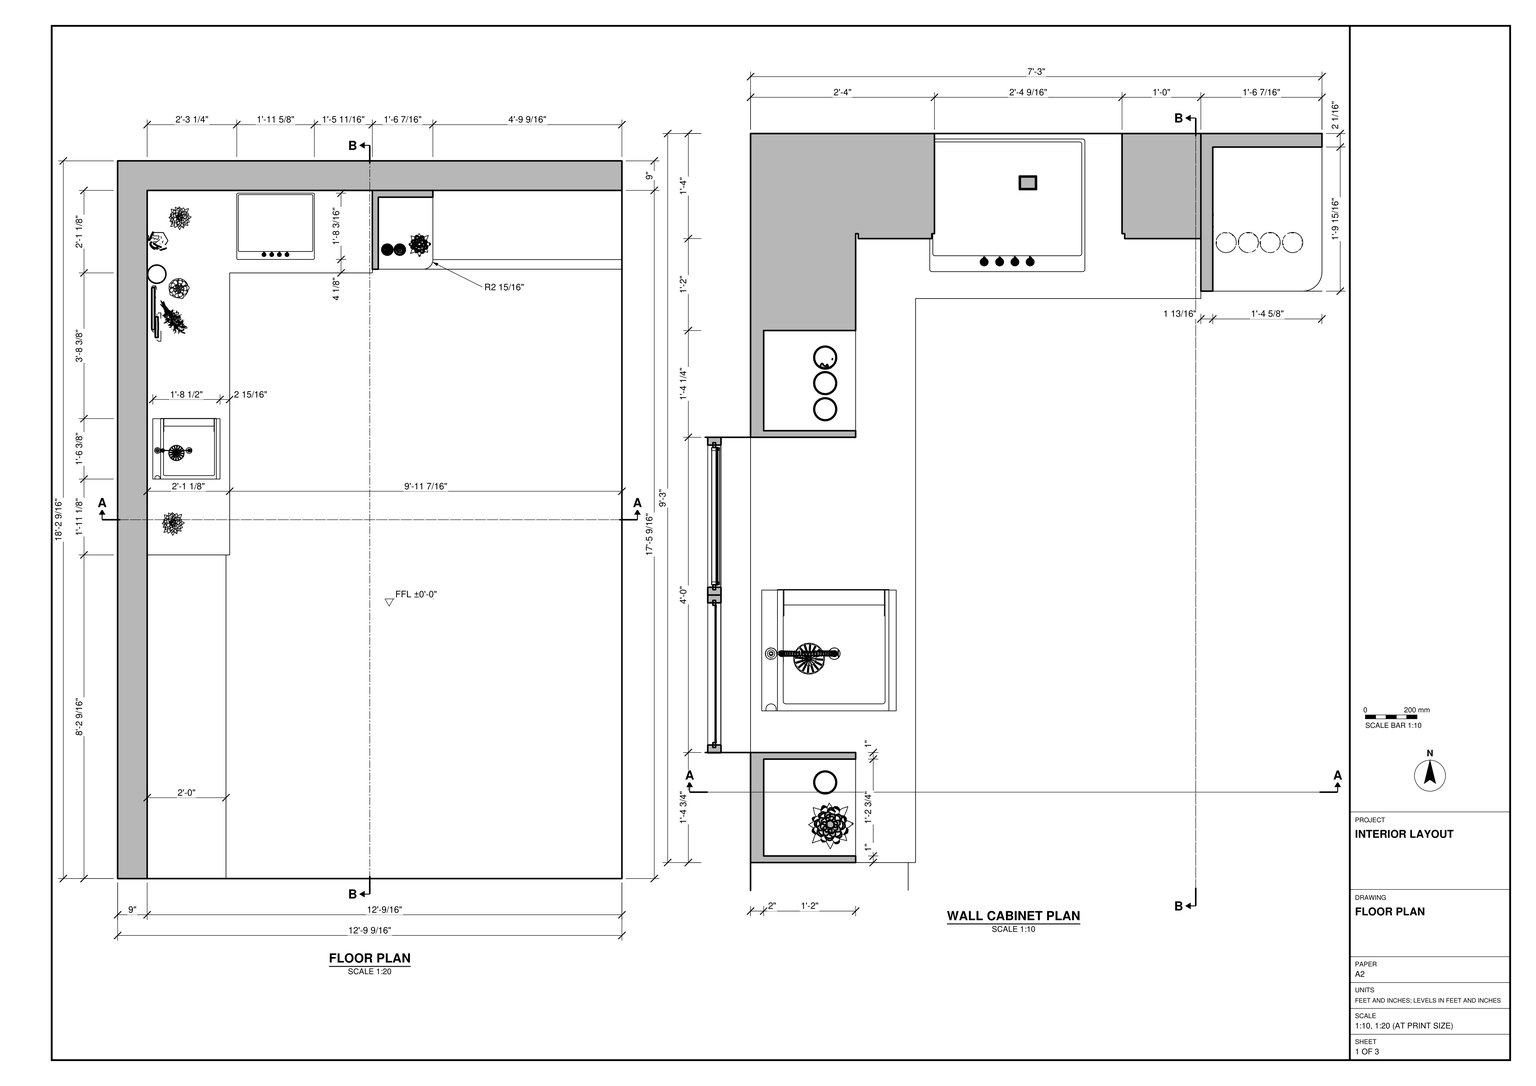
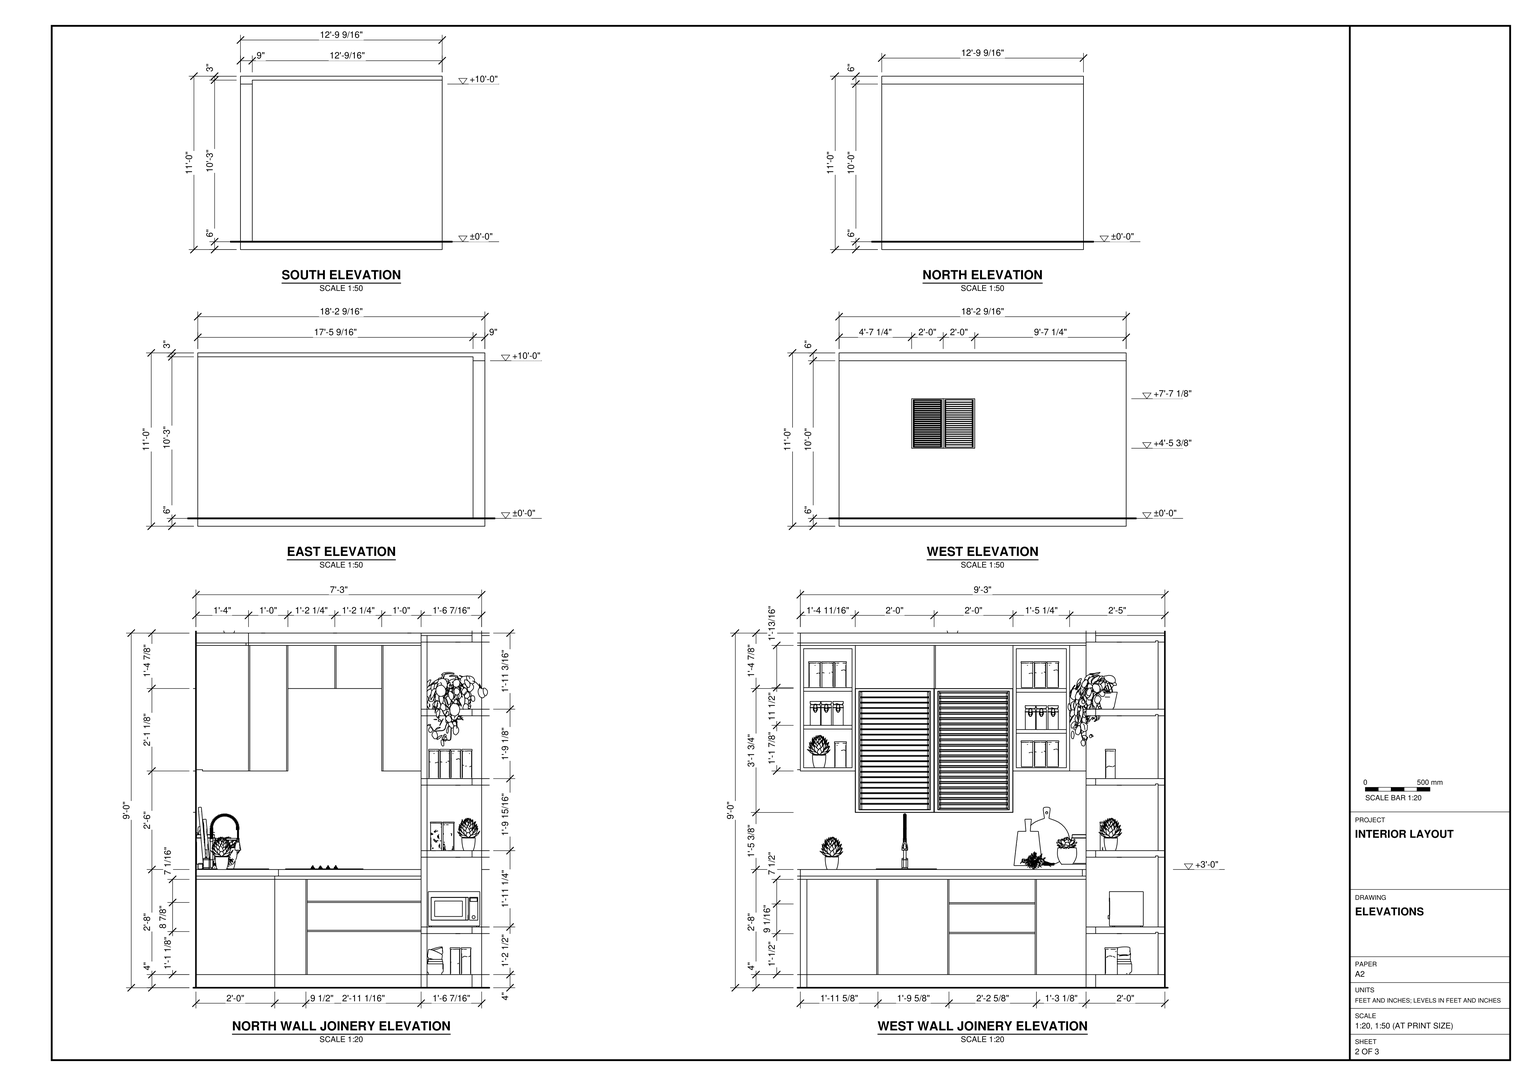
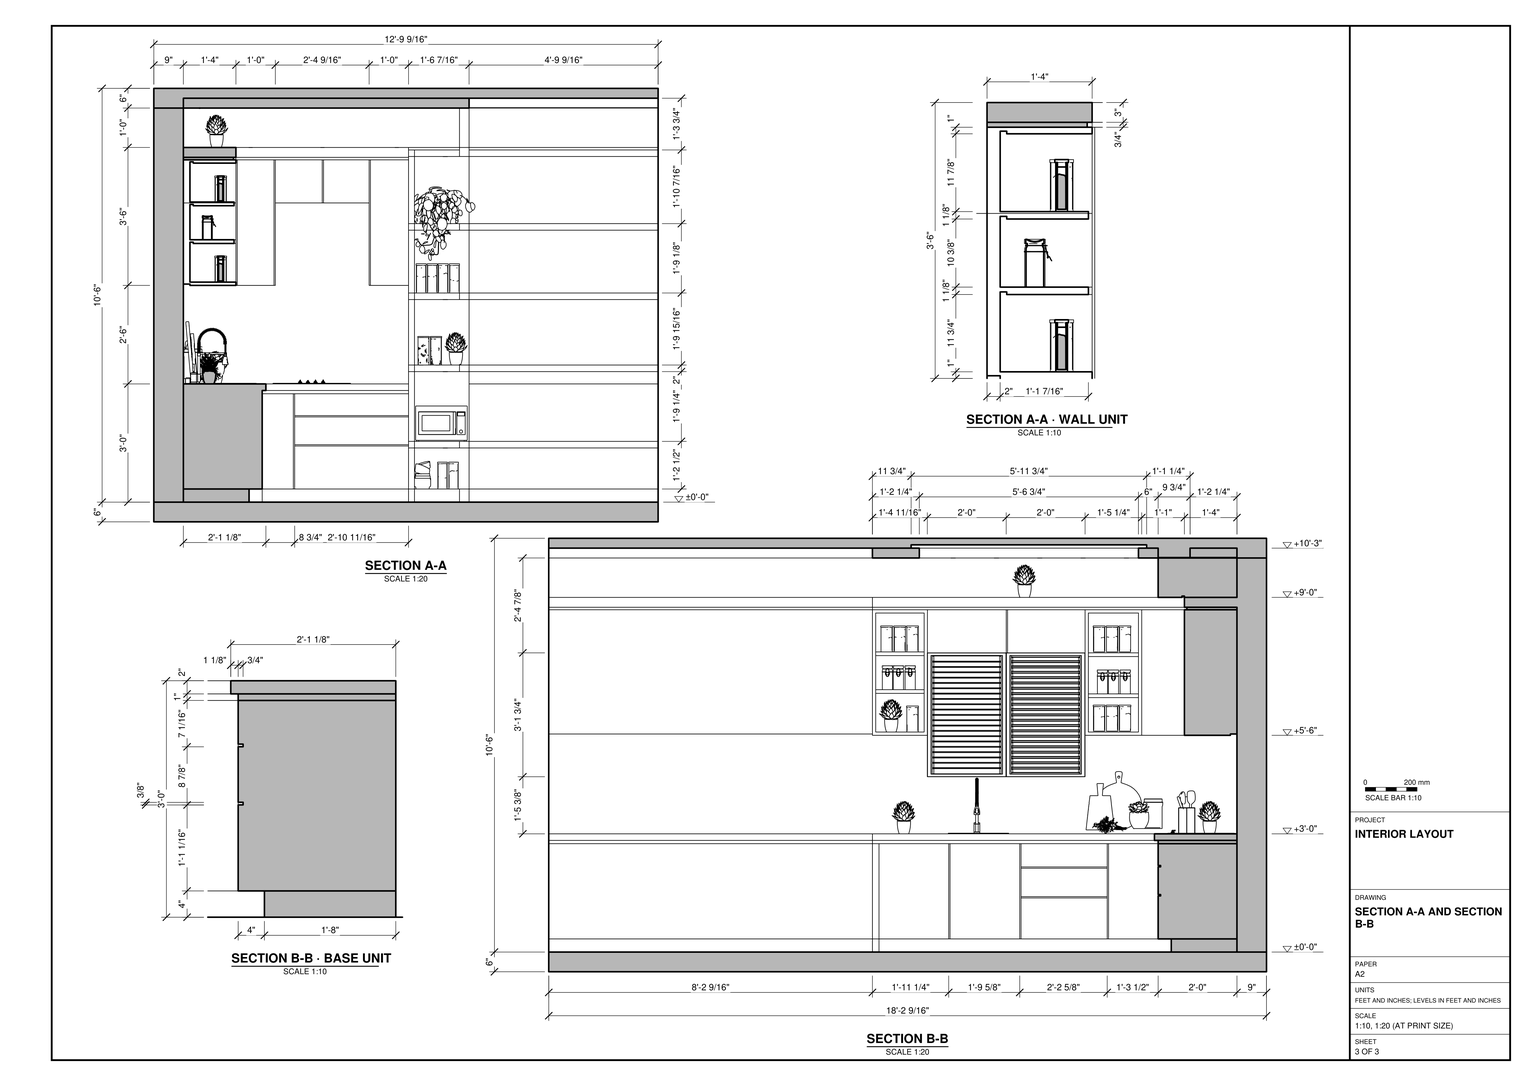
Build the kitchen interior in SketchUp using task_files/diagram_01.pdf. Work in feet and inches. Set the finished floor level to ±0'-0". The overall model measures 12'-9 9/16" east to west, 18'-2 9/16" north to south and 11'-0" high. Model the floor slab, the 9" north and west walls, and the overhead slab, using the sections to establish their vertical relationships. Keep the south and east sides open as drawn.

Fit the kitchen into the northwest corner, leaving the floor in front of the cabinets clear. Use the floor plan to position the sink and cooktop and the wall cabinet plan to set out the storage above them. Place the sink and tap below the paired louvred window on the west wall. On the north wall, leave clearance over the cooktop by stepping up the underside of the wall cabinets. Follow the joinery elevations and sections for the worktop depth, recessed plinths, cupboard fronts, drawer divisions and open shelving bays.

Decor and loose items, including plants, containers and appliances, may be any suitable library components. Keep shell elements and individual joinery pieces in separate groups or components, and use components for repeated parts. Save one SketchUp model as output_files/corner_kitchen_with_fitted_cabinets_and_open_shelving.skp.

# SketchUp Ruby script. Lengths in inches.
U = 1.inch
M = Sketchup.active_model
def pt(a) = Geom::Point3d.new(a.map { |v| v * U })
def face(e, loops, mat)
  f = e.add_face(loops[0].map { |a| pt(a) })
  loops[1..].each { |l| e.add_face(l.map { |a| pt(a) }).erase! }
  f.material = f.back_material = mat if mat
  f
end
# faces: each face lists its corners as indices into pts; further lists are holes
def faces(e, pts, list, mat = nil) = list.each { |f| face(e, (f[0].is_a?(Array) ? f : [f]).map { |l| l.map { |i| pts[i] } }, mat) }
# xy, xz, yz: faces in a plane at the given z, y or x. An outline is a flat list of corners, or four numbers for a rectangle; further outlines are holes
def ring(l) = l.size == 4 ? [[l[0], l[1]], [l[2], l[1]], [l[2], l[3]], [l[0], l[3]]] : l.each_slice(2).to_a
def flat(e, list, mat, &to3) = list.each { |f| face(e, (f[0].is_a?(Array) ? f : [f]).map { |l| ring(l).map { |u, v| to3.(u, v) } }, mat) }
def xy(e, z, list, mat = nil) = flat(e, list, mat) { |x, y| [x, y, z] }
def xz(e, y, list, mat = nil) = flat(e, list, mat) { |x, z| [x, y, z] }
def yz(e, x, list, mat = nil) = flat(e, list, mat) { |y, z| [x, y, z] }
def lines(e, pts, list) = list.each { |a, b| e.add_line(pt(pts[a]), pt(pts[b])) }
# prism: a flat outline (further loops are holes) pulled along v
def prism(e, loops, v, mat = nil)
  f = face(e, loops, mat); d = Geom::Vector3d.new(v.map { |x| x * U })
  f.pushpull(f.normal.samedirection?(d) ? d.length : -d.length)
end
def box(e, o, s, mat = nil) = prism(e, [[o, [o[0] + s[0], o[1], o[2]], [o[0] + s[0], o[1] + s[1], o[2]], [o[0], o[1] + s[1], o[2]]]], [0, 0, s[2]], mat)
def at(x, y, z, deg = 0) = Geom::Transformation.translation(pt([x, y, z])) * Geom::Transformation.rotation(ORIGIN, Z_AXIS, deg.degrees)
def axes(o, x, y, z) = Geom::Transformation.new([*x, 0, *y, 0, *z, 0, *pt(o).to_a, 1])
def part(name) = M.definitions.add(name)
# library, detail: a bought-in or finely detailed component or shape, given as its bounding box
def library(name, o, s) = part(name).tap { |d| box(d.entities, o, s) }
def detail(e, o, s) = box(e.add_group.entities, o, s)
def put(e, d, t, mat = nil) = e.add_instance(d, t).tap { |i| i.material = mat if mat }
def group(e, t, mat = nil) = e.add_group.tap { |g| g.transformation = t; g.material = mat if mat }.entities
root = M.entities
M.materials.add("Emissive").color = [211, 212, 165]
M.materials.add("Generic").color = [219, 224, 214]
M.materials.add("Generic\#1").color = [232, 228, 228]
M.materials.add("Marble Black 01 150cm").color = [31, 31, 31]
M.materials.add("Tiles Simple 02 100cm").color = [183, 183, 183]
M.materials.add("[Color M05]").color = [114, 114, 114]
M.materials.add("[Color M06]").color = [86, 86, 86]
M.materials.add("[Color M08]").color = [30, 30, 30]
M.materials.add("[Wood Floor Light]").color = [204, 176, 127]
c1 = library("Chimney",[0,-0.01,0],[29.73,15.52,29.75])
c2 = library("1045",[78.33,40.52,-0.08],[23.62,20.2,1.2])
c3 = library("Utensils",[0,-0.54,-0.24],[6.34,6.28,13.37])
c4 = library("ACCESS \#103",[-1.07,0,-1.17],[14.88,24.44,20.18])
c5 = library("kitchen utensils",[105.73,-44.48,4],[78.44,98.38,95.31])
c6 = library("Potted Plant 50-23",[-3.4,-3.5,0],[6.8,7,9.93])
c7 = library("Peperomia 450 001",[-6.6875,-10.1875,-9.42],[16.7,12.74,19.03])
c8 = library("JSilva Jalousie",[-31.89,-0.05,0.1],[63.78,4.97,70.86])
c9 = library("sink",[-18.39,0,-10.63],[18.4,20.47,27.45])
c10 = library("Tlon Light 1950 Ceiling 152 010",[-38.39,-38.39,-3.78],[76.78,76.78,3.41])
c11 = library("Microwave 10-11",[-10.28,-7.99,0],[20.56,15.98,13.07])
xy(root,-6,[[0,0,153.5625,218.5625]])
xy(root,0,[[0,0,9,0,9,209.5625,153.5625,209.5625,153.5625,218.5625,0,218.5625],[9,0,33,98.5625],[9,98.5625,33,98.5625,33,100.5625,29,100.5625,29,189.5625,33,189.5625,33,209.5625,9,209.5625],[77.5625,185.5625,93.07,185.5625,93.46,185.59,93.83,185.66,94.19,185.79,94.54,185.95,94.86,186.17,95.14,186.42,95.4,186.71,95.61,187.03,95.78,187.37,95.9,187.73,95.97,188.11,96,188.49,96,209.5625,77.5625,209.5625],[93.07,185.5625,153.5625,185.5625,153.5625,188.49,96,188.49,95.97,188.11,95.9,187.73,95.78,187.37,95.61,187.03,95.4,186.71,95.14,186.42,94.86,186.17,94.54,185.95,94.19,185.79,93.83,185.66,93.46,185.59],
  [96,188.49,153.5625,209.5625],[33,189.5625,77.5625,209.5625]])
xy(root,0,[[33,0,153.5625,0,153.5625,185.5625,77.5625,185.5625,77.5625,189.5625,29,189.5625,29,100.5625,33,100.5625]],"Tiles Simple 02 100cm")
xy(root,4,[[9,98.5625,33,100.5625],[9,100.5625,9,209.5625,33,209.5625,33,189.5625,29,189.5625,29,100.5625],[29,122.1875,33,143.42],[77.5625,185.5625,77.5625,209.5625,96,209.5625,96,207.5,79.375,207.5,79.375,185.5625],[42.49,186.3125,42.89,189.5625],
  [33,189.5625,77.5625,209.5625]])
xy(root,4,[[29,100.5625,33,121.79],[29,121.79,32.25,122.1875],[29,143.42,32.25,143.82],[29,143.82,33,170.06],[29,170.06,32.25,170.46],
  [29,170.46,33,189.5625],[33,185.5625,42.49,189.5625],[42.89,185.5625,77.5625,189.5625]],"[Color M05]")
xy(root,4,[[79.375,185.5625,79.375,207.5,96,207.5,96,188.49,95.97,188.11,95.9,187.73,95.78,187.37,95.61,187.03,95.4,186.71,95.14,186.42,94.86,186.17,94.54,185.95,94.19,185.79,93.83,185.66,93.46,185.59,93.07,185.5625]],"[Wood Floor Light]")
xy(root,16.47,[[32.25,143.82,33,170.06]],"[Color M05]")
xy(root,16.5,[[79.375,185.5625,79.375,206.75,96,206.75,96,188.49,95.97,188.11,95.9,187.73,95.78,187.37,95.61,187.03,95.4,186.71,95.14,186.42,94.86,186.17,94.54,185.95,94.19,185.79,93.83,185.66,93.46,185.59,93.07,185.5625]],"[Wood Floor Light]")
xy(root,16.87,[[32.25,143.82,33,170.06]],"[Color M05]")
xy(root,16.9,[[79.375,206.75,96,207.5]],"Emissive")
xy(root,17.1,[[42.89,185.5625,77.5625,186.3125]],"[Color M05]")
xy(root,17.5,[[42.89,185.5625,77.5625,186.3125]],"[Color M05]")
xy(root,18.5,[[79.375,185.5625,93.07,185.5625,93.46,185.59,93.83,185.66,94.19,185.79,94.54,185.95,94.86,186.17,95.14,186.42,95.4,186.71,95.61,187.03,95.78,187.37,95.9,187.73,95.97,188.11,96,188.49,96,207.5,79.375,207.5]],"[Wood Floor Light]")
xy(root,25.52,[[32.25,143.82,33,170.06]],"[Color M05]")
xy(root,25.625,[[13.1,121.66,30.0625,140.14]])
xy(root,25.92,[[32.25,143.82,33,170.06]],"[Color M05]")
xy(root,25.96,[[42.89,185.5625,77.5625,186.3125]],"[Color M05]")
xy(root,26.36,[[42.89,185.5625,77.5625,186.3125]],"[Color M05]")
xy(root,33,[[9,98.5625,33,100.5625],[33,185.5625,33,209.5625,77.5625,209.5625,77.5625,185.5625,42.89,185.5625,42.89,186.3125,42.49,186.3125,42.49,185.5625]])
xy(root,33,[[32.25,121.79,33,122.1875],[32.25,143.42,33,143.82],[32.25,170.06,33,170.46],[42.49,185.5625,42.89,186.3125]],"[Color M05]")
xy(root,34,[[33,185.5625,77.5625,209.5625]])
xy(root,34,[[33,98.5625,34.125,185.5625],[34.125,184.4375,77.5625,185.5625]],"Marble Black 01 150cm")
xy(root,36,[[[9,98.5625,34.125,98.5625,34.125,184.4375,77.5625,184.4375,77.5625,209.5625,9,209.5625],[13.1,121.66,30.0625,140.14]]],"Marble Black 01 150cm")
xy(root,39.75,[[79.375,185.5625,79.375,206.75,96,206.75,96,188.49,95.97,188.11,95.9,187.73,95.78,187.37,95.61,187.03,95.4,186.71,95.14,186.42,94.86,186.17,94.54,185.95,94.19,185.79,93.83,185.66,93.46,185.59,93.07,185.5625]],"[Wood Floor Light]")
xy(root,40.15,[[79.375,206.75,96,207.5]],"Emissive")
xy(root,41.75,[[79.375,185.5625,93.07,185.5625,93.46,185.59,93.83,185.66,94.19,185.79,94.54,185.95,94.86,186.17,95.14,186.42,95.4,186.71,95.61,187.03,95.78,187.37,95.9,187.73,95.97,188.11,96,188.49,96,207.5,79.375,207.5]],"[Wood Floor Light]")
xy(root,53.42,[[0,115.3125,9,163.3125]],"Marble Black 01 150cm")
xy(root,61.6875,[[79.375,185.5625,79.375,206.75,96,206.75,96,188.49,95.97,188.11,95.9,187.73,95.78,187.37,95.61,187.03,95.4,186.71,95.14,186.42,94.86,186.17,94.54,185.95,94.19,185.79,93.83,185.66,93.46,185.59,93.07,185.5625]],"[Wood Floor Light]")
xy(root,62.09,[[79.375,206.75,96,207.5]],"Emissive")
xy(root,63.6875,[[79.375,185.5625,93.07,185.5625,93.46,185.59,93.83,185.66,94.19,185.79,94.54,185.95,94.86,186.17,95.14,186.42,95.4,186.71,95.61,187.03,95.78,187.37,95.9,187.73,95.97,188.11,96,188.49,96,207.5,79.375,207.5]],"[Wood Floor Light]")
xy(root,66,[[11,98.5625,25,115.3125],[11,163.3125,11,207.5625,37,207.5625,37,194.3125,36.6,194.3125,36.6,193.5625,25.4,193.5625,25.4,194.3125,25,194.3125,25,163.3125],[65.96,193.5625,65.96,194.3125,65.5625,194.3125,65.5625,207.5625,77.5625,207.5625,77.5625,193.5625]],"Generic")
xy(root,66.4,[[9,98.5625,11,115.3125],[9,163.3125,9,209.5625,37,209.5625,37,207.5625,11,207.5625,11,163.3125],[65.5625,207.5625,77.5625,209.5625]],"Emissive")
xy(root,67,[[11,99.5625,25,114.3125],[11,164.3125,25,179.57]],"[Wood Floor Light]")
xy(root,77.48,[[12,164.3125,24.4375,179.57]],"[Wood Floor Light]")
xy(root,77.88,[[11,164.3125,12,179.57]],"Emissive")
xy(root,78.61,[[11,164.3125,24.4375,179.57]])
xy(root,78.77,[[12,99.5625,24.4375,114.3125]],"[Wood Floor Light]")
xy(root,79.17,[[11,99.5625,12,114.3125]],"Emissive")
xy(root,79.9,[[11,99.5625,24.4375,114.3125]],"[Wood Floor Light]")
xy(root,82.8125,[[79.375,185.5625,79.375,206.75,96,206.75,96,188.49,95.97,188.11,95.9,187.73,95.78,187.37,95.61,187.03,95.4,186.71,95.14,186.42,94.86,186.17,94.54,185.95,94.19,185.79,93.83,185.66,93.46,185.59,93.07,185.5625]],"[Wood Floor Light]")
xy(root,83.21,[[79.375,206.75,96,207.5]],"Emissive")
xy(root,84.8125,[[79.375,185.5625,93.07,185.5625,93.46,185.59,93.83,185.66,94.19,185.79,94.54,185.95,94.86,186.17,95.14,186.42,95.4,186.71,95.61,187.03,95.78,187.37,95.9,187.73,95.97,188.11,96,188.49,96,207.5,79.375,207.5]],"[Wood Floor Light]")
xy(root,89.98,[[12,164.3125,24.4375,179.57]],"[Wood Floor Light]")
xy(root,90.27,[[12,99.5625,24.4375,114.3125]],"[Wood Floor Light]")
xy(root,90.38,[[11,164.3125,12,179.57]],"Emissive")
xy(root,90.67,[[11,99.5625,12,114.3125]],"Emissive")
xy(root,91.11,[[0,115.3125,9,163.3125]])
xy(root,91.11,[[9,115.3125,9,163.3125,25,163.3125,25,139.71,24.25,139.71,24.25,139.3125,25,139.3125,25,115.3125],[37,193.5625,37,209.5625,65.5625,209.5625,65.5625,193.5625,51.68,193.5625,51.68,194.3125,51.28,194.3125,51.28,193.5625]],"Generic")
xy(root,91.11,[[11,164.3125,24.4375,179.57]],"[Wood Floor Light]")
xy(root,91.4,[[11,99.5625,24.4375,114.3125]],"[Wood Floor Light]")
xy(root,103.24,[[12,99.5625,25,114.3125],[12,164.3125,25,179.57]],"[Wood Floor Light]")
xy(root,103.64,[[11,99.5625,12,114.3125],[11,164.3125,12,179.57]],"Emissive")
xy(root,104.24,[[9,98.5625,24.25,115.3125],[9,115.3125,24.25,163.3125],[9,163.3125,24.25,193.5625],[9,193.5625,9,209.5625,25,209.5625,25,194.3125,24.25,194.3125,24.25,193.5625],[25,194.3125,37,209.5625],
  [37,194.3125,65.5625,209.5625],[65.5625,194.3125,77.5625,209.5625]])
xy(root,104.24,[[24.25,98.5625,25,115.3125],[24.25,115.3125,25,139.3125],[24.25,139.71,25,163.3125],[24.25,163.3125,25,180.57],[24.25,180.57,25,193.5625],
  [24.25,193.5625,25,194.3125],[25.4,193.5625,36.6,194.3125],[37,193.5625,51.28,194.3125],[51.68,193.5625,65.5625,194.3125],[65.96,193.5625,77.5625,194.3125]],"[Color M05]")
xy(root,104.99,[[9,98.5625,24.25,98.5625,24.25,194.3125,25,194.3125,25,209.5625,9,209.5625],[25,194.3125,77.5625,209.5625]])
xy(root,104.99,[[24.25,98.5625,25,194.3125],[25,193.5625,77.5625,194.3125]],"[Color M05]")
xy(root,105.25,[[79.375,185.5625,79.375,206.75,96,206.75,96,188.49,95.97,188.11,95.9,187.73,95.78,187.37,95.61,187.03,95.4,186.71,95.14,186.42,94.86,186.17,94.54,185.95,94.19,185.79,93.83,185.66,93.46,185.59,93.07,185.5625]],"[Wood Floor Light]")
xy(root,105.65,[[79.375,206.75,96,207.5]],"Emissive")
xy(root,107.25,[[77.5625,185.5625,93.07,186.3125]],"[Color M05]")
xy(root,108,[[9,185.5625,25,209.5625],[93.07,185.5625,93.07,186.3125,77.5625,186.3125,77.5625,209.5625,96,209.5625,96,188.49,95.97,188.11,95.9,187.73,95.78,187.37,95.61,187.03,95.4,186.71,95.14,186.42,94.86,186.17,94.54,185.95,94.19,185.79,93.83,185.66,93.46,185.59],[25,193.5625,77.5625,209.5625]])
xy(root,108,[[25,185.5625,77.5625,192.8125],[77.5625,185.5625,93.07,186.3125]],"[Color M05]")
xy(root,108,[[9,98.5625,25,185.5625]],"[Color M06]")
xy(root,108.4,[[25,192.8125,77.5625,193.5625]],"Emissive")
xy(root,120,[[0,0,0,218.5625,153.5625,218.5625,153.5625,209.5625,9,209.5625,9,0],[23.28,185.5625,81.72,195.28]])
xy(root,120,[[[9,98.5625,9,185.5625,81.72,185.5625,81.72,195.28,23.28,195.28,23.28,185.5625,9,185.5625,9,209.5625,96,209.5625,96,98.5625],[23.28,112.84,81.72,179.5625]]],"Generic\#1")
xy(root,120.125,[[9,185.5625,93.07,185.5625,93.46,185.59,93.83,185.66,94.19,185.79,94.54,185.95,94.86,186.17,95.14,186.42,95.4,186.71,95.61,187.03,95.78,187.37,95.9,187.73,95.97,188.11,96,188.49,96,209.5625,9,209.5625]])
xy(root,123,[[9,0,153.5625,98.5625],[[9,98.5625,9,185.5625,81.72,185.5625,81.72,195.28,23.28,195.28,23.28,185.5625,9,185.5625,9,209.5625,96,209.5625,96,98.5625],[20.78,110.34,84.22,182.0625]],[96,98.5625,153.5625,188.49],[96,188.49,153.5625,209.5625]])
xy(root,123,[[20.78,110.34,23.28,182.0625],[23.28,110.34,84.22,112.84],[81.72,112.84,84.22,179.5625],[23.28,179.5625,84.22,182.0625]],"Emissive")
xy(root,124,[[20.78,110.34,84.22,182.0625]],"Generic\#1")
xy(root,126,[[0,0,153.5625,218.5625]])
xz(root,0,[[0,-6,153.5625,0],[0,0,9,120],[9,0,153.5625,123],[0,120,9,120,9,123,153.5625,123,153.5625,126,0,126]])
xz(root,98.5625,[[9,120,96,123]])
xz(root,98.5625,[[9,4,33,33],[11,66,25,66,25,104.24,9,104.24,9,66.4,11,66.4]],"Generic")
xz(root,98.5625,[[9,34,34.125,36]],"Marble Black 01 150cm")
xz(root,98.5625,[[9,0,33,4],[9,33,33,34],[9,104.24,24.25,104.99],[9,104.99,25,108]],"[Color M05]")
xz(root,99.5625,[[24.4375,78.77,25,79.9]])
xz(root,99.5625,[[11,67,11,79.17,12,79.17,12,78.77,25,78.77,25,67],[11,79.9,11,90.67,12,90.67,12,90.27,24.4375,90.27,24.4375,91.4,11,91.4,11,103.64,12,103.64,12,103.24,25,103.24,25,79.9]],"[Wood Floor Light]")
xz(root,100.5625,[[9,4,33,33]])
xz(root,100.5625,[[29,0,33,4]],"[Color M05]")
xz(root,110.34,[[20.78,123,84.22,124]],"Emissive")
xz(root,112.84,[[23.28,120,81.72,123]])
xz(root,114.3125,[[11,67,25,67,25,78.77,12,78.77,12,79.17,11,79.17],[24.4375,78.77,25,79.9],[11,79.9,25,79.9,25,91.11,24.4375,91.11,24.4375,90.27,12,90.27,12,90.67,11,90.67],[24.4375,91.11,25,91.11,25,103.24,12,103.24,12,103.64,11,103.64,11,91.4,24.4375,91.4]],"[Wood Floor Light]")
xz(root,115.3125,[[11,66,11,66.4,9,66.4,9,91.11,25,91.11,25,66],[9,91.11,25,104.24]])
xz(root,115.3125,[[0,53.42,9,66],[0,66,9,91.11]],"Marble Black 01 150cm")
xz(root,121.66,[[13.1,25.625,30.0625,36]])
xz(root,121.79,[[32.25,4,33,33]],"[Color M05]")
xz(root,122.1875,[[32.25,4,33,33]],"[Color M05]")
xz(root,139.3125,[[24.25,91.11,25,104.24]],"[Color M05]")
xz(root,139.71,[[24.25,91.11,25,104.24]],"[Color M05]")
xz(root,140.14,[[13.1,25.625,30.0625,36]])
xz(root,143.42,[[32.25,4,33,33]],"[Color M05]")
xz(root,143.82,[[32.25,4,33,16.47],[32.25,16.87,33,25.52],[32.25,25.92,33,33]],"[Color M05]")
xz(root,163.3125,[[9,91.11,25,104.24]])
xz(root,163.3125,[[11,66,25,66,25,91.11,9,91.11,9,66.4,11,66.4]],"Generic")
xz(root,163.3125,[[0,53.42,9,66],[0,66,9,91.11]],"Marble Black 01 150cm")
xz(root,164.3125,[[12,77.48,12,77.88,11,77.88,11,78.61,24.4375,78.61,24.4375,77.48],[12,89.98,12,90.38,11,90.38,11,91.11,24.4375,91.11,24.4375,89.98]])
xz(root,164.3125,[[11,67,11,77.88,12,77.88,12,77.48,24.4375,77.48,24.4375,78.61,11,78.61,11,90.38,12,90.38,12,89.98,24.4375,89.98,24.4375,91.11,25,91.11,25,67],[11,91.11,11,103.64,12,103.64,12,103.24,25,103.24,25,91.11]],"[Wood Floor Light]")
xz(root,170.06,[[32.25,4,33,16.47],[32.25,16.87,33,25.52],[32.25,25.92,33,33]],"[Color M05]")
xz(root,170.46,[[32.25,4,33,33]],"[Color M05]")
xz(root,179.5625,[[23.28,120,81.72,123]],"Generic\#1")
xz(root,179.57,[[12,77.48,24.4375,77.48,24.4375,78.61,11,78.61,11,77.88,12,77.88],[12,89.98,24.4375,89.98,24.4375,91.11,11,91.11,11,90.38,12,90.38]])
xz(root,179.57,[[11,67,25,67,25,103.24,12,103.24,12,103.64,11,103.64,11,91.11,24.4375,91.11,24.4375,89.98,12,89.98,12,90.38,11,90.38,11,78.61,24.4375,78.61,24.4375,77.48,12,77.48,12,77.88,11,77.88]],"[Wood Floor Light]")
xz(root,182.0625,[[20.78,123,84.22,124]],"Emissive")
xz(root,184.4375,[[34.125,34,77.5625,36]],"Marble Black 01 150cm")
xz(root,185.5625,[[9,120,23.28,120.125],[23.28,120,81.72,120.125],[81.72,120,93.07,120.125],[9,120.125,23.28,123],[23.28,120.125,81.72,123]])
xz(root,185.5625,[[33,4,42.49,33],[42.89,4,77.5625,17.1],[42.89,17.5,77.5625,25.96],[42.89,26.36,77.5625,33]],"Generic")
xz(root,185.5625,[[77.5625,0,79.375,4],[79.375,0,93.07,4],[77.5625,4,79.375,16.5],[77.5625,16.5,79.375,18.5],[79.375,16.5,93.07,18.5],
  [77.5625,18.5,79.375,39.75],[33,33,77.5625,34],[77.5625,39.75,79.375,41.75],[79.375,39.75,93.07,41.75],[77.5625,41.75,79.375,61.6875],
  [77.5625,61.6875,79.375,63.6875],[79.375,61.6875,93.07,63.6875],[77.5625,63.6875,79.375,82.8125],[77.5625,82.8125,79.375,84.8125],[79.375,82.8125,93.07,84.8125],
  [77.5625,84.8125,79.375,105.25],[77.5625,105.25,79.375,107.25],[79.375,105.25,93.07,107.25],[9,108,93.07,120]],"[Color M05]")
xz(root,186.3125,[[42.49,4,42.89,33],[42.89,17.1,77.5625,17.5],[42.89,25.96,77.5625,26.36],[77.5625,107.25,93.07,108]],"[Color M05]")
xz(root,189.5625,[[29,0,33,4],[33,0,77.5625,4]],"[Color M05]")
xz(root,192.8125,[[25,108,77.5625,108.4]],"Emissive")
xz(root,193.5625,[[25,108,77.5625,108.4]],"Emissive")
xz(root,193.5625,[[25.4,66,36.6,104.24],[65.96,66,77.5625,104.24],[37,91.11,51.28,104.24],[51.68,91.11,65.5625,104.24]],"Generic")
xz(root,193.5625,[[25,104.99,77.5625,108]],"[Color M05]")
xz(root,194.3125,[[25,66,25.4,104.24],[36.6,66,37,104.24],[65.5625,66,65.96,104.24],[51.28,91.11,51.68,104.24],[24.25,104.24,25,104.99],
  [25,104.24,77.5625,104.99]],"[Color M05]")
xz(root,195.28,[[23.28,120,81.72,123]])
xz(root,206.75,[[79.375,16.5,96,16.9],[79.375,39.75,96,40.15],[79.375,61.6875,96,62.09],[79.375,82.8125,96,83.21],[79.375,105.25,96,105.65]],"Emissive")
xz(root,207.5,[[79.375,4,96,16.9],[79.375,18.5,96,40.15],[79.375,41.75,96,62.09],[79.375,63.6875,96,83.21],[79.375,84.8125,96,105.65]],"[Wood Floor Light]")
xz(root,207.5625,[[11,66,37,66.4],[65.5625,66,77.5625,66.4]],"Emissive")
xz(root,209.5625,[[9,0,33,4],[33,0,77.5625,4],[77.5625,0,96,4],[96,0,153.5625,4],[9,4,33,33],
  [33,4,77.5625,33],[77.5625,4,96,36],[96,4,153.5625,16.5],[96,16.5,153.5625,18.5],[96,18.5,153.5625,36],
  [9,33,33,36],[33,33,77.5625,34],[33,34,77.5625,36],[77.5625,36,96,108],[96,36,153.5625,39.75],
  [96,39.75,153.5625,41.75],[96,41.75,153.5625,61.6875],[96,61.6875,153.5625,63.6875],[96,63.6875,153.5625,82.8125],[9,66.4,25,104.24],
  [25,66.4,37,104.24],[65.5625,66.4,77.5625,104.24],[96,82.8125,153.5625,84.8125],[96,84.8125,153.5625,105.25],[37,91.11,65.5625,104.24],
  [9,104.24,25,104.99],[25,104.24,77.5625,104.99],[9,104.99,25,108],[96,105.25,153.5625,107.25],[96,107.25,153.5625,108],
  [9,108,96,120],[96,108,153.5625,120],[9,120,96,120.125],[96,120,153.5625,120.125],[9,120.125,96,123],
  [96,120.125,153.5625,123]])
xz(root,209.5625,[[9,36,77.5625,36,77.5625,66.4,65.5625,66.4,65.5625,91.11,37,91.11,37,66.4,9,66.4]],"Marble Black 01 150cm")
xz(root,218.5625,[[0,-6,153.5625,0],[0,0,153.5625,120],[0,120,153.5625,126]])
yz(root,0,[[0,-6,218.5625,0],[[0,0,218.5625,120],[115.3125,53.42,163.3125,91.11]],[0,120,218.5625,126]])
yz(root,9,[[0,0,98.5625,4],[98.5625,0,209.5625,4],[0,4,98.5625,33],[98.5625,4,100.5625,33],[100.5625,4,209.5625,33],
  [0,33,98.5625,34],[98.5625,33,209.5625,36],[0,34,98.5625,36],[0,66.4,98.5625,104.24],[98.5625,66.4,115.3125,104.24],
  [163.3125,66.4,193.5625,104.24],[193.5625,66.4,209.5625,104.24],[115.3125,91.11,163.3125,104.24],[0,104.24,98.5625,104.99],[98.5625,104.24,209.5625,104.99],
  [0,104.99,98.5625,108],[98.5625,104.99,209.5625,108],[185.5625,108,209.5625,120],[0,120,98.5625,123],[98.5625,120,185.5625,123],
  [185.5625,120,209.5625,120.125],[185.5625,120.125,209.5625,123]])
yz(root,9,[[0,108,185.5625,120]],"Generic\#1")
yz(root,9,[[0,36,209.5625,36,209.5625,66.4,163.3125,66.4,163.3125,53.42,115.3125,53.42,115.3125,66.4,0,66.4]],"Marble Black 01 150cm")
yz(root,11,[[164.3125,77.88,179.57,78.61],[164.3125,90.38,179.57,91.11]])
yz(root,11,[[98.5625,66,115.3125,66.4],[163.3125,66,207.5625,66.4]],"Emissive")
yz(root,11,[[99.5625,67,114.3125,79.17],[164.3125,67,179.57,77.88],[164.3125,78.61,179.57,90.38],[99.5625,79.9,114.3125,90.67],[164.3125,91.11,179.57,103.64],
  [99.5625,91.4,114.3125,103.64]],"[Wood Floor Light]")
yz(root,12,[[164.3125,77.48,179.57,77.88],[99.5625,78.77,114.3125,79.17],[164.3125,89.98,179.57,90.38],[99.5625,90.27,114.3125,90.67],[99.5625,103.24,114.3125,103.64],
  [164.3125,103.24,179.57,103.64]],"Emissive")
yz(root,13.1,[[121.66,25.625,140.14,36]])
yz(root,20.78,[[110.34,123,182.0625,124]],"Emissive")
yz(root,23.28,[[185.5625,120,195.28,123]])
yz(root,23.28,[[112.84,120,179.5625,123]],"Generic\#1")
yz(root,24.25,[[139.3125,91.11,139.71,104.24],[98.5625,104.24,194.3125,104.99]],"[Color M05]")
yz(root,24.4375,[[164.3125,77.48,179.57,78.61],[99.5625,78.77,114.3125,79.9],[164.3125,89.98,179.57,91.11],[99.5625,90.27,114.3125,91.4]],"[Wood Floor Light]")
yz(root,25,[[194.3125,104.24,209.5625,104.99],[193.5625,104.99,209.5625,108]])
yz(root,25,[[192.8125,108,193.5625,108.4]],"Emissive")
yz(root,25,[[180.57,66,193.5625,104.24],[115.3125,91.11,139.3125,104.24],[139.71,91.11,163.3125,104.24]],"Generic")
yz(root,25,[[[98.5625,66,115.3125,104.24],[99.5625,67,114.3125,103.24]],[[163.3125,66,180.57,104.24],[164.3125,67,179.57,103.24]],[193.5625,66,194.3125,104.24],[98.5625,104.99,193.5625,108]],"[Color M05]")
yz(root,25.4,[[193.5625,66,194.3125,104.24]],"[Color M05]")
yz(root,29,[[100.5625,0,189.5625,4]],"[Color M05]")
yz(root,30.0625,[[121.66,25.625,140.14,36]])
yz(root,32.25,[[121.79,4,122.1875,33],[143.42,4,143.82,33],[170.06,4,170.46,33],[143.82,16.47,170.06,16.87],[143.82,25.52,170.06,25.92]],"[Color M05]")
yz(root,33,[[189.5625,0,209.5625,4],[185.5625,4,209.5625,33],[185.5625,33,209.5625,34]])
yz(root,33,[[100.5625,4,121.79,33],[122.1875,4,143.42,33],[143.82,4,170.06,16.47],[170.46,4,185.5625,33],[143.82,16.87,170.06,25.52],
  [143.82,25.92,170.06,33]],"Generic")
yz(root,33,[[98.5625,0,100.5625,4],[98.5625,4,100.5625,33],[98.5625,33,185.5625,34]],"[Color M05]")
yz(root,34.125,[[98.5625,34,184.4375,36]],"Marble Black 01 150cm")
yz(root,36.6,[[193.5625,66,194.3125,91.11],[193.5625,91.11,194.3125,104.24]],"[Color M05]")
yz(root,37,[[194.3125,91.11,209.5625,104.24]])
yz(root,37,[[194.3125,66,207.5625,66,207.5625,66.4,209.5625,66.4,209.5625,91.11,194.3125,91.11]],"Generic")
yz(root,37,[[193.5625,91.11,194.3125,104.24]],"[Color M05]")
yz(root,42.49,[[185.5625,4,186.3125,33]],"[Color M05]")
yz(root,42.89,[[185.5625,4,186.3125,17.1],[185.5625,17.5,186.3125,25.96],[185.5625,26.36,186.3125,33]],"[Color M05]")
yz(root,51.28,[[193.5625,91.11,194.3125,104.24]],"[Color M05]")
yz(root,51.68,[[193.5625,91.11,194.3125,104.24]],"[Color M05]")
yz(root,65.5625,[[194.3125,66,194.3125,91.11,209.5625,91.11,209.5625,66.4,207.5625,66.4,207.5625,66],[194.3125,91.11,209.5625,104.24]])
yz(root,65.5625,[[193.5625,91.11,194.3125,104.24]],"[Color M05]")
yz(root,65.96,[[193.5625,66,194.3125,91.11],[193.5625,91.11,194.3125,104.24]],"[Color M05]")
yz(root,77.5625,[[189.5625,0,209.5625,4],[185.5625,4,185.5625,17.1,186.3125,17.1,186.3125,17.5,185.5625,17.5,185.5625,25.96,186.3125,25.96,186.3125,26.36,185.5625,26.36,185.5625,33,209.5625,33,209.5625,4],[185.5625,33,209.5625,34],[184.4375,34,185.5625,36],[185.5625,34,209.5625,36],
  [193.5625,66,193.5625,104.24,209.5625,104.24,209.5625,66.4,207.5625,66.4,207.5625,66],[194.3125,104.24,209.5625,104.99],[193.5625,104.99,209.5625,108]])
yz(root,77.5625,[[192.8125,108,193.5625,108.4]],"Emissive")
yz(root,77.5625,[[185.5625,0,189.5625,4],[185.5625,17.1,186.3125,17.5],[185.5625,25.96,186.3125,26.36],[185.5625,36,185.5625,107.25,186.3125,107.25,186.3125,108,193.5625,108,193.5625,104.99,194.3125,104.99,194.3125,104.24,193.5625,104.24,193.5625,66,207.5625,66,207.5625,66.4,209.5625,66.4,209.5625,36]],"[Color M05]")
yz(root,79.375,[[185.5625,4,207.5,4,207.5,16.9,206.75,16.9,206.75,16.5,185.5625,16.5],[185.5625,18.5,207.5,18.5,207.5,40.15,206.75,40.15,206.75,39.75,185.5625,39.75],[185.5625,41.75,207.5,41.75,207.5,62.09,206.75,62.09,206.75,61.6875,185.5625,61.6875],[185.5625,63.6875,207.5,63.6875,207.5,83.21,206.75,83.21,206.75,82.8125,185.5625,82.8125],[185.5625,84.8125,207.5,84.8125,207.5,105.65,206.75,105.65,206.75,105.25,185.5625,105.25]],"[Wood Floor Light]")
yz(root,81.72,[[185.5625,120,188.49,123],[188.49,120,195.28,123]])
yz(root,81.72,[[112.84,120,179.5625,123]],"Generic\#1")
yz(root,84.22,[[110.34,123,182.0625,124]],"Emissive")
yz(root,93.07,[[185.5625,107.25,186.3125,108]])
yz(root,96,[[98.5625,120,188.49,123],[188.49,120,209.5625,120.125],[188.49,120.125,209.5625,123]])
yz(root,96,[[188.49,0,209.5625,4],[207.5,4,209.5625,16.5],[188.49,16.5,206.75,16.5,206.75,16.9,207.5,16.9,207.5,16.5,209.5625,16.5,209.5625,18.5,188.49,18.5],[207.5,18.5,209.5625,39.75],[188.49,39.75,206.75,39.75,206.75,40.15,207.5,40.15,207.5,39.75,209.5625,39.75,209.5625,41.75,188.49,41.75],
  [207.5,41.75,209.5625,61.6875],[188.49,61.6875,206.75,61.6875,206.75,62.09,207.5,62.09,207.5,61.6875,209.5625,61.6875,209.5625,63.6875,188.49,63.6875],[207.5,63.6875,209.5625,82.8125],[188.49,82.8125,206.75,82.8125,206.75,83.21,207.5,83.21,207.5,82.8125,209.5625,82.8125,209.5625,84.8125,188.49,84.8125],[207.5,84.8125,209.5625,105.25],
  [188.49,105.25,206.75,105.25,206.75,105.65,207.5,105.65,207.5,105.25,209.5625,105.25,209.5625,107.25,188.49,107.25],[188.49,107.25,209.5625,108],[188.49,108,209.5625,120]],"[Color M05]")
yz(root,153.5625,[[0,-6,218.5625,0],[0,0,209.5625,123],[209.5625,0,218.5625,120],[209.5625,120,218.5625,120,218.5625,126,0,126,0,123,209.5625,123]])
p = [[93.07,185.5625,4],[93.46,185.59,4],[93.46,185.59,0],[93.07,185.5625,0],[93.83,185.66,4],[93.83,185.66,0],
  [94.19,185.79,4],[94.19,185.79,0],[94.54,185.95,4],[94.54,185.95,0],[94.86,186.17,4],[94.86,186.17,0],
  [95.14,186.42,4],[95.14,186.42,0],[95.4,186.71,4],[95.4,186.71,0],[95.61,187.03,4],[95.61,187.03,0],
  [95.78,187.37,4],[95.78,187.37,0],[95.9,187.73,4],[95.9,187.73,0],[95.97,188.11,4],[95.97,188.11,0],
  [96,188.49,4],[96,188.49,0],[93.46,185.59,18.5],[93.07,185.5625,18.5],[93.07,185.5625,16.5],[93.46,185.59,16.5],
  [93.83,185.66,18.5],[93.83,185.66,16.5],[94.19,185.79,18.5],[94.19,185.79,16.5],[94.54,185.95,18.5],[94.54,185.95,16.5],
  [94.86,186.17,18.5],[94.86,186.17,16.5],[95.14,186.42,18.5],[95.14,186.42,16.5],[95.4,186.71,18.5],[95.4,186.71,16.5],
  [95.61,187.03,18.5],[95.61,187.03,16.5],[95.78,187.37,18.5],[95.78,187.37,16.5],[95.9,187.73,18.5],[95.9,187.73,16.5],
  [95.97,188.11,18.5],[95.97,188.11,16.5],[96,188.49,18.5],[96,188.49,16.5],[93.46,185.59,41.75],[93.07,185.5625,41.75],
  [93.07,185.5625,39.75],[93.46,185.59,39.75],[93.83,185.66,41.75],[93.83,185.66,39.75],[94.19,185.79,41.75],[94.19,185.79,39.75],
  [94.54,185.95,41.75],[94.54,185.95,39.75],[94.86,186.17,41.75],[94.86,186.17,39.75],[95.14,186.42,41.75],[95.14,186.42,39.75],
  [95.4,186.71,41.75],[95.4,186.71,39.75],[95.61,187.03,41.75],[95.61,187.03,39.75],[95.78,187.37,41.75],[95.78,187.37,39.75],
  [95.9,187.73,41.75],[95.9,187.73,39.75],[95.97,188.11,41.75],[95.97,188.11,39.75],[96,188.49,41.75],[96,188.49,39.75],
  [93.46,185.59,63.6875],[93.07,185.5625,63.6875],[93.07,185.5625,61.6875],[93.46,185.59,61.6875],[93.83,185.66,63.6875],[93.83,185.66,61.6875],
  [94.19,185.79,63.6875],[94.19,185.79,61.6875],[94.54,185.95,63.6875],[94.54,185.95,61.6875],[94.86,186.17,63.6875],[94.86,186.17,61.6875],
  [95.14,186.42,63.6875],[95.14,186.42,61.6875],[95.4,186.71,63.6875],[95.4,186.71,61.6875],[95.61,187.03,63.6875],[95.61,187.03,61.6875],
  [95.78,187.37,63.6875],[95.78,187.37,61.6875],[95.9,187.73,63.6875],[95.9,187.73,61.6875],[95.97,188.11,63.6875],[95.97,188.11,61.6875],
  [96,188.49,63.6875],[96,188.49,61.6875],[93.46,185.59,84.8125],[93.07,185.5625,84.8125],[93.07,185.5625,82.8125],[93.46,185.59,82.8125],
  [93.83,185.66,84.8125],[93.83,185.66,82.8125],[94.19,185.79,84.8125],[94.19,185.79,82.8125],[94.54,185.95,84.8125],[94.54,185.95,82.8125],
  [94.86,186.17,84.8125],[94.86,186.17,82.8125],[95.14,186.42,84.8125],[95.14,186.42,82.8125],[95.4,186.71,84.8125],[95.4,186.71,82.8125],
  [95.61,187.03,84.8125],[95.61,187.03,82.8125],[95.78,187.37,84.8125],[95.78,187.37,82.8125],[95.9,187.73,84.8125],[95.9,187.73,82.8125],
  [95.97,188.11,84.8125],[95.97,188.11,82.8125],[96,188.49,84.8125],[96,188.49,82.8125],[93.07,185.5625,105.25],[93.46,185.59,105.25],
  [93.46,185.59,108],[93.07,185.5625,108],[93.07,185.5625,107.25],[93.83,185.66,105.25],[93.83,185.66,108],[94.19,185.79,105.25],
  [94.19,185.79,108],[94.54,185.95,105.25],[94.54,185.95,108],[94.86,186.17,105.25],[94.86,186.17,108],[95.14,186.42,105.25],
  [95.14,186.42,108],[95.4,186.71,105.25],[95.4,186.71,108],[95.61,187.03,105.25],[95.61,187.03,108],[95.78,187.37,105.25],
  [95.78,187.37,108],[95.9,187.73,105.25],[95.9,187.73,108],[95.97,188.11,105.25],[95.97,188.11,108],[96,188.49,105.25],
  [96,188.49,107.25],[96,188.49,108],[93.46,185.59,120.125],[93.07,185.5625,120.125],[93.07,185.5625,120],[93.83,185.66,120.125],
  [94.19,185.79,120.125],[94.54,185.95,120.125],[94.86,186.17,120.125],[95.14,186.42,120.125],[95.4,186.71,120.125],[95.61,187.03,120.125],
  [95.78,187.37,120.125],[95.9,187.73,120.125],[95.97,188.11,120.125],[96,188.49,120.125],[96,188.49,120]]
faces(root,p,[[0,1,2,3],[1,4,5,2],[4,6,7,5],[6,8,9,7],[8,10,11,9],[10,12,13,11],[12,14,15,13],[14,16,17,15],
  [16,18,19,17],[18,20,21,19],[20,22,23,21],[22,24,25,23],[26,27,28,29],[30,26,29,31],[32,30,31,33],[34,32,33,35],
  [36,34,35,37],[38,36,37,39],[40,38,39,41],[42,40,41,43],[44,42,43,45],[46,44,45,47],[48,46,47,49],[50,48,49,51],
  [52,53,54,55],[56,52,55,57],[58,56,57,59],[60,58,59,61],[62,60,61,63],[64,62,63,65],[66,64,65,67],[68,66,67,69],
  [70,68,69,71],[72,70,71,73],[74,72,73,75],[76,74,75,77],[78,79,80,81],[82,78,81,83],[84,82,83,85],[86,84,85,87],
  [88,86,87,89],[90,88,89,91],[92,90,91,93],[94,92,93,95],[96,94,95,97],[98,96,97,99],[100,98,99,101],[102,100,101,103],
  [104,105,106,107],[108,104,107,109],[110,108,109,111],[112,110,111,113],[114,112,113,115],[116,114,115,117],[118,116,117,119],[120,118,119,121],
  [122,120,121,123],[124,122,123,125],[126,124,125,127],[128,126,127,129],[130,131,132,133,134],[131,135,136,132],[135,137,138,136],[137,139,140,138],
  [139,141,142,140],[141,143,144,142],[143,145,146,144],[145,147,148,146],[147,149,150,148],[149,151,152,150],[151,153,154,152],[153,155,156,157,154],
  [158,159,160,133,132],[161,158,132,136],[162,161,136,138],[163,162,138,140],[164,163,140,142],[165,164,142,144],[166,165,144,146],[167,166,146,148],
  [168,167,148,150],[169,168,150,152],[170,169,152,154],[171,170,154,157,172]],"[Color M05]")
put(root,c1,axes([37,193.57,72.07],[0.96075,0,0],[0,1,0],[0,0,0.64]))
put(root,c2,at(-42.05,148.01,36.08))
put(root,c3,at(9,191.36,36))
put(root,c4,at(9,163.62,36))
put(root,c5,at(-91.09,145.57,0))
put(root,c6,at(16.93,108,36))
put(root,c6,at(21.24,104.14,67))
put(root,c6,at(19.15,144.75,108))
put(root,c6,at(92.04,192.93,41.75))
put(root,c6,at(19,201.1,36))
put(root,c7,axes([85.99,192.05,84.7],[1.18,0,0],[0,1.18,0],[0,0,1.18]))
put(root,c8,axes([4.5,139.29,53.33],[0,0.75323,0],[-0.41,0,0],[0,0,0.53249]))
put(root,c9,at(31.18,140.05,36.2,90))
put(root,c10,axes([73.98,188.29,108.03],[0.01464,0,0],[0,0.01464,0],[0,0,0.01464]))
put(root,c10,axes([51.36,188.29,108.03],[0.01464,0,0],[0,0.01464,0],[0,0,0.01464]))
put(root,c10,axes([29.48,188.29,108.03],[0.01464,0,0],[0,0.01464,0],[0,0,0.01464]))
put(root,c10,axes([88.75,195.68,105.28],[0.01801,0,0],[0,0.01801,0],[0,0,0.01801]))
put(root,c10,axes([88.75,195.68,82.84],[0.01801,0,0],[0,0.01801,0],[0,0,0.01801]))
put(root,c10,axes([88.75,195.68,61.71],[0.01801,0,0],[0,0.01801,0],[0,0,0.01801]))
put(root,c10,axes([88.75,195.68,39.78],[0.01801,0,0],[0,0.01801,0],[0,0,0.01801]))
put(root,c10,axes([88.75,195.68,16.53],[0.01801,0,0],[0,0.01801,0],[0,0,0.01801]))
put(root,c10,axes([13.96,175.9,120.03],[0.01801,0,0],[0,0.01801,0],[0,0,0.01801]))
put(root,c10,axes([13.96,162.71,120.03],[0.01801,0,0],[0,0.01801,0],[0,0,0.01801]))
put(root,c10,axes([13.96,149.52,120.03],[0.01801,0,0],[0,0.01801,0],[0,0,0.01801]))
put(root,c10,axes([13.96,136.33,120.03],[0.01801,0,0],[0,0.01801,0],[0,0,0.01801]))
put(root,c10,axes([13.96,123.15,120.03],[0.01801,0,0],[0,0.01801,0],[0,0,0.01801]))
put(root,c10,axes([13.96,109.96,120.03],[0.01801,0,0],[0,0.01801,0],[0,0,0.01801]))
put(root,c11,axes([87.59,197.64,18.5],[0.76467,0,0],[0,0.67,0],[0,0,0.8241]),"[Color M08]")
